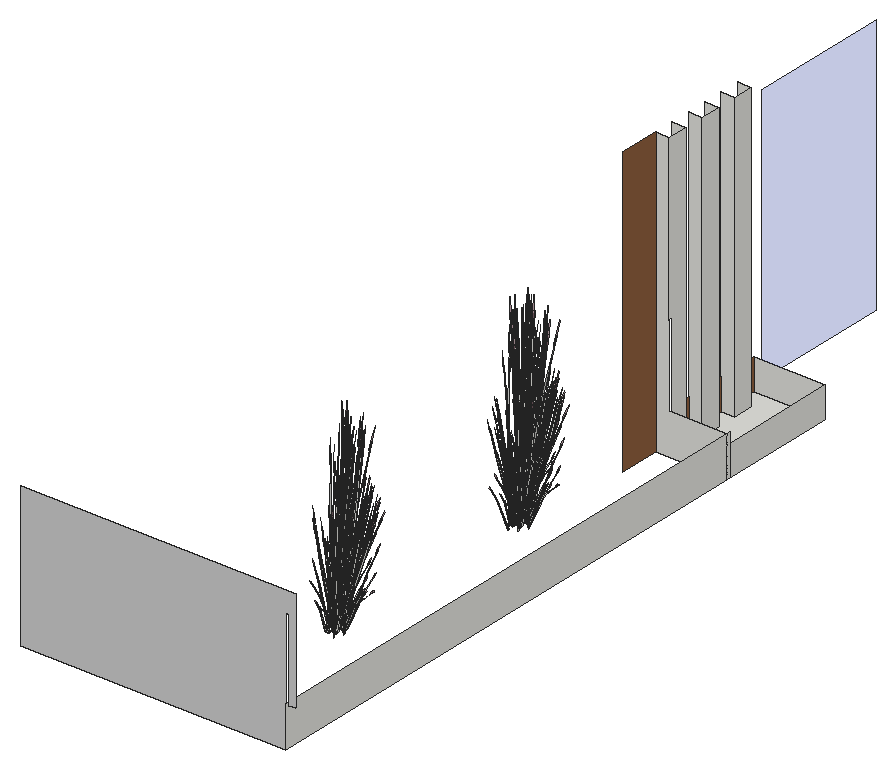
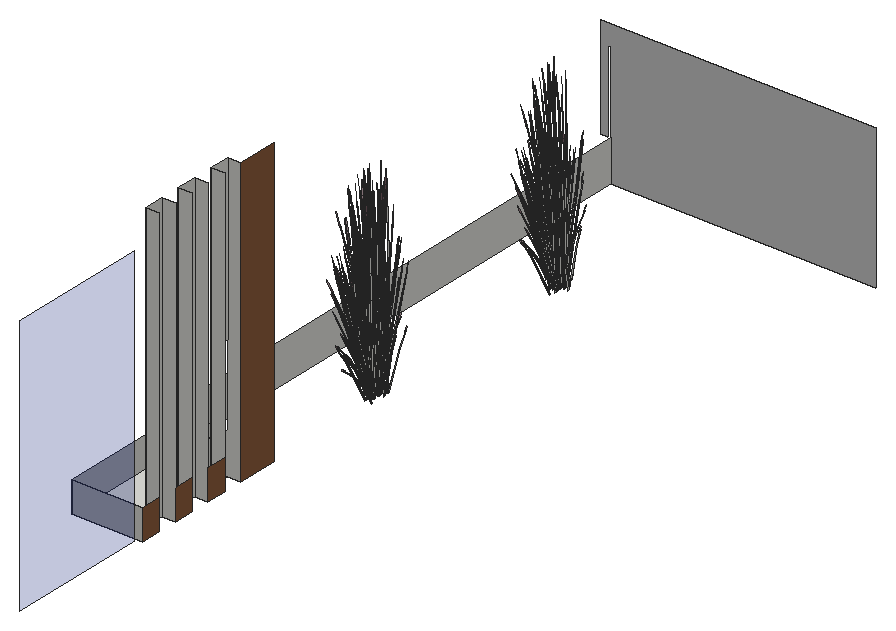
# SketchUp Ruby script. Lengths in inches.
U = 1.inch
M = Sketchup.active_model
def pt(a) = Geom::Point3d.new(a.map { |v| v * U })
def face(e, loops, mat)
  f = e.add_face(loops[0].map { |a| pt(a) })
  loops[1..].each { |l| e.add_face(l.map { |a| pt(a) }).erase! }
  f.material = f.back_material = mat if mat
  f
end
# faces: each face lists its corners as indices into pts; further lists are holes
def faces(e, pts, list, mat = nil) = list.each { |f| face(e, (f[0].is_a?(Array) ? f : [f]).map { |l| l.map { |i| pts[i] } }, mat) }
# xy, xz, yz: faces in a plane at the given z, y or x. An outline is a flat list of corners, or four numbers for a rectangle; further outlines are holes
def ring(l) = l.size == 4 ? [[l[0], l[1]], [l[2], l[1]], [l[2], l[3]], [l[0], l[3]]] : l.each_slice(2).to_a
def flat(e, list, mat, &to3) = list.each { |f| face(e, (f[0].is_a?(Array) ? f : [f]).map { |l| ring(l).map { |u, v| to3.(u, v) } }, mat) }
def xy(e, z, list, mat = nil) = flat(e, list, mat) { |x, y| [x, y, z] }
def xz(e, y, list, mat = nil) = flat(e, list, mat) { |x, z| [x, y, z] }
def yz(e, x, list, mat = nil) = flat(e, list, mat) { |y, z| [x, y, z] }
def lines(e, pts, list) = list.each { |a, b| e.add_line(pt(pts[a]), pt(pts[b])) }
# prism: a flat outline (further loops are holes) pulled along v
def prism(e, loops, v, mat = nil)
  f = face(e, loops, mat); d = Geom::Vector3d.new(v.map { |x| x * U })
  f.pushpull(f.normal.samedirection?(d) ? d.length : -d.length)
end
def box(e, o, s, mat = nil) = prism(e, [[o, [o[0] + s[0], o[1], o[2]], [o[0] + s[0], o[1] + s[1], o[2]], [o[0], o[1] + s[1], o[2]]]], [0, 0, s[2]], mat)
def at(x, y, z, deg = 0) = Geom::Transformation.translation(pt([x, y, z])) * Geom::Transformation.rotation(ORIGIN, Z_AXIS, deg.degrees)
def axes(o, x, y, z) = Geom::Transformation.new([*x, 0, *y, 0, *z, 0, *pt(o).to_a, 1])
def part(name) = M.definitions.add(name)
# library, detail: a bought-in or finely detailed component or shape, given as its bounding box
def library(name, o, s) = part(name).tap { |d| box(d.entities, o, s) }
def detail(e, o, s) = box(e.add_group.entities, o, s)
def put(e, d, t, mat = nil) = e.add_instance(d, t).tap { |i| i.material = mat if mat }
def group(e, t, mat = nil) = e.add_group.tap { |g| g.transformation = t; g.material = mat if mat }.entities
root = M.entities
M.materials.add("Glass_Basic_01").color = [23, 48, 186]
M.materials["Glass_Basic_01"].alpha = 0.25
M.materials.add("LightPink_Translucent").color = [144, 107, 117]
M.materials["LightPink_Translucent"].alpha = 0.75
M.materials.add("Wood_Veneer_15_1K").color = [142, 95, 62]
M.materials.add("[Cladding_Siding_White]1").color = [207, 207, 207]
c1 = part("blade")
p = [[2.15,0.21,22],[0,0.17,0],[0.09,0.45,0],[2.18,0.31,22],[2.29,0.31,22],[0.38,0.45,0],
  [2.48,0.24,33],[2.49,0.24,33],[2.48,0.22,33]]
faces(c1.entities,p,[[0,1,2,3],[4,5,2,3],[6,3,4,7],[8,0,3,6]])
c2 = part("seeds")
p = [[0.3,-0.1,1.38],[-0.01,-0.03,1.59],[-0.01,-0.03,0.03],[0.14,-0.07,-0.07],[0.29,-0.03,3],[0.15,0.01,3.11]]
faces(c2.entities,p,[[0,1,2,3],[1,0,4,5]],"LightPink_Translucent")
c3 = part("blade with seeds")
put(c3.entities,c1,at(0,0,0))
put(c3.entities,c2,axes([2.4,0.25,30.99],[1.5799,-0.05474,1.17369],[-0.12525,1.92788,0.29478],[-0.07173,-0.02425,1.56792]))
xy(root,402,[[364,255,381,256],[364,256,381,256,381,291,360,291,360,285,364,285,364,279,360,279,360,273,364,273,364,267,360,267,360,261,364,261]])
xz(root,93,[[303,402,303,444,384,444,384,414,382,414,382,438,381,438,381,402]],"[Cladding_Siding_White]1")
xz(root,255,[[360,402,381,402,381,414,364,414,364,486,360,486]])
xz(root,256,[[364,402,381,411]])
xz(root,261,[[360,402,364,486]])
xz(root,267,[[360,402,364,486]])
xz(root,273,[[360,402,364,486]])
xz(root,279,[[360,402,364,486]])
xz(root,285,[[360,402,364,486]])
xz(root,291,[[360,402,381,411]])
yz(root,360,[[294,403.5,336,480]],"Glass_Basic_01")
yz(root,360,[[243,402,255,486],[261,402,267,411],[273,402,279,411],[285,402,291,411]],"Wood_Veneer_15_1K")
yz(root,364,[[256,402,261,402,261,486,255,486,255,438,256,438],[267,402,273,486],[279,402,285,486]])
yz(root,381,[[93,402,255,414],[255,402,256,414],[256,402,291,411]])
put(root,c3,axes([357.37,140.09,404.33],[-0.52621,0.16023,0.16584],[-0.12993,-0.59629,0.32981],[0.04693,0.08688,1.50782]))
put(root,c3,axes([356.83,137.86,404.6],[0.06282,0.35202,1.07969],[-0.34848,-0.19497,0.79328],[0.0375,-0.18025,0.23781]))
put(root,c3,axes([356.6,145.46,407.31],[0.3384,-0.34633,-0.06098],[0.31006,0.3793,-0.27651],[0.02183,0.10747,0.91203]))
put(root,c3,axes([356.51,140.96,404.22],[-0.40602,0.54785,0.43009],[-0.48237,-0.48361,0.16877],[0.09788,-0.05467,1.49325]))
put(root,c3,axes([357.2,141.82,404.08],[0.34183,0.38994,0],[-0.34183,0.38994,0],[0,0,1.5911]))
put(root,c3,axes([357.7,208.44,404.33],[0.52621,-0.16023,0.16584],[0.12993,0.59629,0.32981],[-0.04693,-0.08688,1.50782]))
put(root,c3,axes([357.2,141.37,404.56],[0.23759,-0.54397,0.42055],[0.49367,0.26179,-0.2024],[0,0.12539,1.35025]))
put(root,c3,axes([356.99,143.26,404.07],[0.49367,0.27103,0],[-0.23759,0.56315,0],[0,0,1.64456]))
put(root,c3,axes([358.375,208.54,404.0625],[-0.49367,-0.27103,0],[0.23759,-0.56315,0],[0,0,1.52945]))
put(root,c3,axes([358.75,204.62,406.75],[-0.14763,0.46424,0.33289],[-0.4307,-0.1354,-0.42977],[-0.03949,-0.18691,0.82232]))
put(root,c3,axes([359.52,209.22,404.23],[0.30616,0.60492,0],[-0.51222,0.33735,-0.48511],[-0.11666,0.07683,1.53889]))
put(root,c3,axes([356.29,143.98,406.4],[0.48137,0.15133,-0.48033],[-0.165,0.51886,-0.37205],[0.04414,0.2089,0.91906]))
put(root,c3,axes([355.88,144,406.73],[0.47919,-0.28106,-0.11431],[0.23549,0.49884,-0.63445],[0.06322,0.21021,0.96403]))
put(root,c3,axes([357.04,141.24,404.24],[-0.61893,-0.12719,0.46247],[0.12596,-0.71835,0.18148],[0.09045,0.06936,1.60565]))
put(root,c3,axes([357.96,209.48,406.76],[-0.48252,-0.15782,0.50086],[0.165,-0.51886,0.41298],[0.029,0.20404,1.03641]))
put(root,c3,axes([358.33,138.43,406.43],[-0.04973,0.04611,1.6674],[-0.48725,-0.15557,-0.15755],[-0.01764,-0.20123,0.29507]))
put(root,c3,axes([357.94,139.76,406.73],[-0.53819,-0.02991,-0.11431],[0.01471,-0.56632,-0.63445],[0.03738,-0.21811,0.96403]))
put(root,c3,axes([358.45,142.22,403.91],[-0.34183,0.37665,-0.29119],[-0.34183,-0.37665,0.29119],[0,0.12132,1.30635]))
put(root,c3,axes([357.83,209.52,406.45],[-0.36083,0.20517,0.06044],[-0.17661,-0.37413,0.47584],[0.03485,0.16492,0.72558]))
put(root,c3,axes([359.27,208.48,404.33],[0.14146,-0.59996,0.16584],[0.51766,0.16978,0.32981],[-0.08942,0.00292,1.50782]))
put(root,c3,axes([359.03,207.68,404.46],[0.36178,0.36271,0.13611],[-0.30177,0.40921,-0.38866],[-0.084,0.05532,1.1914]))
put(root,c3,axes([357.47,142.15,403.97],[0.17956,0.55272,-0.65059],[-0.51723,0.19906,-0.17075],[0.01985,0.18717,1.43607]))
put(root,c3,axes([357.22,141.56,404.07],[0.54787,0,0],[0,0.62498,0],[0,0,1.67702]))
put(root,c3,axes([358.9,207.23,404.16],[-0.45549,-0.5196,-0.05763],[0.45577,-0.51991,0],[-0.01591,-0.01814,1.65037]))
put(root,c3,axes([357.73,139.85,406.75],[-0.33133,0.31784,0.33289],[-0.31365,-0.36292,-0.42977],[0.04772,-0.1844,0.82232]))
put(root,c3,axes([359.02,207.42,404.56],[0.53176,-0.03727,0.42055],[0.04809,0.6186,-0.2024],[-0.0952,0.0627,1.35025]))
put(root,c3,axes([356.6875,140.87,404.56],[-0.29417,-0.5067,0.42055],[0.44558,-0.35681,-0.2024],[0.0952,0.0627,1.35025]))
put(root,c3,axes([356.15,140.99,404.51],[-0.05706,-0.68884,-0.2735],[0.59432,-0.04165,-0.47002],[0.10465,-0.09176,1.50125]))
put(root,c3,axes([357.41,141.49,404.46],[0.45625,-0.17605,0.13611],[0.15978,0.50273,-0.38866],[0,0.11064,1.1914]))
put(root,c3,axes([357.58,139.55,406.4],[-0.35055,-0.40562,-0.48033],[0.37031,-0.35523,-0.37205],[0.05334,-0.20609,0.91906]))
put(root,c3,axes([359.15,208.84,404.19],[0.61306,0.19622,0.28911],[-0.15337,0.70136,-0.34302],[-0.10147,0.08778,1.54992]))
put(root,c3,axes([358.25,203.46,403.4],[-0.08214,0.02175,1.65762],[-0.45422,-0.24483,-0.25323],[0.00762,-0.20421,0.28235]))
put(root,c3,axes([359.41,208.8,404.33],[0.4583,-0.30184,0.46672],[0.27394,0.54125,0],[-0.10438,0.06875,1.48054]))
put(root,c3,axes([358.7,204.13,406.25],[0.14763,-0.46424,-0.33289],[0.4307,0.1354,0.42977],[-0.03949,-0.18691,0.82232]))
put(root,c3,axes([357.98,206.64,404.22],[0.2129,0.67504,0.43009],[-0.60833,0.23474,0.16877],[0.00743,-0.12404,1.49325]))
put(root,c3,axes([357.25,141.53,404.51],[0.55148,0.28805,-0.2735],[-0.26554,0.60796,-0.47002],[0.01733,0.14927,1.50125]))
put(root,c3,axes([357.88,206.55,404.08],[0.23759,-0.54397,-0.42055],[0.49367,0.26179,0.2024],[0,-0.12539,1.35025]))
put(root,c3,axes([358.49,208.3,404.07],[-0.15978,-0.52046,0],[0.45625,-0.18226,0],[0,0,1.45109]))
put(root,c3,axes([357.91,209.4,403.4],[0.07925,-0.03285,1.65762],[0.47671,0.18081,-0.25323],[0.01394,0.20378,0.28235]))
put(root,c3,axes([356.07,139.46,403.91],[0.45686,0.14937,-0.29119],[-0.11503,0.52602,0.29119],[0.0921,-0.06066,1.30635]))
put(root,c3,axes([358.01,209.59,406.25],[-0.14763,0.46424,-0.33289],[-0.4307,-0.1354,0.42977],[0.03949,0.18691,0.82232]))
put(root,c3,axes([357.35,138.83,404.44],[-0.13919,0.12219,1.34422],[-0.41687,-0.21387,-0.28909],[0.07727,-0.26598,0.57472]))
put(root,c3,axes([358.45,141.67,404.33],[0,-0.60368,0.46672],[0.54787,0,0],[0,0.13749,1.48054]))
put(root,c3,axes([358.68,142.23,403.9],[0,0.60368,-0.46672],[-0.54787,0,0],[0,0.13749,1.48054]))
put(root,c3,axes([357.22,144.0625,406.45],[-0.48705,0.13854,0.45122],[-0.08453,-0.54345,0.37205],[0.11455,0.16017,0.9337]))
put(root,c3,axes([355.97,139.22,403.9],[0.4583,-0.30184,-0.46672],[0.27394,0.54125,0],[0.10438,-0.06875,1.48054]))
put(root,c3,axes([357.125,144.17,406.45],[-0.22256,0.38349,0.06044],[-0.31694,-0.22327,0.47584],[0.10247,0.12295,0.72558]))
put(root,c3,axes([356.5625,142.9,405.64],[-0.11194,-0.19382,1.61094],[0.51725,-0.16318,0.13026],[0.1169,0.30428,0.68866]))
put(root,c3,axes([356.89,140.73,404.46],[0.09447,-0.53876,0.13611],[0.46155,0.09352,-0.38866],[0.084,0.05532,1.1914]))
put(root,c3,axes([359.13,207.28,404.08],[-0.23759,0.54397,-0.42055],[-0.49367,-0.26179,0.2024],[0,0.12539,1.35025]))
put(root,c3,axes([358.88,204.2,406.45],[0.36083,-0.20517,0.06044],[0.17661,0.37413,0.47584],[-0.03485,-0.16492,0.72558]))
put(root,c3,axes([357.71,210.41,406.43],[0.06207,0.09721,1.64448],[0.50093,0.03819,-0.26007],[0.05037,0.21439,0.13189]))
put(root,c3,axes([357.54,139.79,404.33],[-0.4583,-0.30184,0.46672],[0.27394,-0.54125,0],[0.10438,0.06875,1.48054]))
put(root,c3,axes([360.07,206.95,404.33],[-0.38474,-0.43973,0.16584],[0.38772,-0.42651,0.32981],[-0.04249,0.0898,1.50782]))
put(root,c3,axes([357.68,139.73,406.68],[0.01274,-0.55841,-0.66783],[0.53656,0.0375,0.08059],[0.05662,-0.23657,0.9447]))
put(root,c3,axes([358.74,206.69,404.07],[0,-0.69851,0],[0.61233,0,0],[0,0,1.68689]))
put(root,c3,axes([358.75,204.24,406.45],[0.48252,0.15782,0.45122],[-0.165,0.51886,0.37205],[-0.029,-0.20404,0.9337]))
put(root,c3,axes([358.18,206.82,404.29],[0.55175,0.29259,0.22621],[-0.26554,0.60796,0.47002],[0,-0.14015,1.5091]))
put(root,c3,axes([359.05,206.97,404.15],[0,0.69816,-0.05299],[-0.61233,0,0],[0,0.02194,1.68606]))
put(root,c3,axes([358,206.41,404.56],[-0.53176,0.03727,0.42055],[-0.04809,-0.6186,-0.2024],[0.0952,-0.0627,1.35025]))
put(root,c3,axes([357.14,142.9375,404.05],[0.51411,-0.20483,-0.18046],[0.18065,0.59003,0.00007],[0.05675,-0.02264,1.63463]))
put(root,c3,axes([357.97,209.1,406.75],[0.14763,-0.46424,0.33289],[0.4307,0.1354,-0.42977],[0.03949,0.18691,0.82232]))
put(root,c3,axes([357.75,205.35,404.33],[-0.14146,0.59996,0.16584],[-0.51766,-0.16978,0.32981],[0.08942,-0.00292,1.50782]))
put(root,c3,axes([358.76,208.32,404.15],[0.2129,0.69353,-0.05652],[-0.60833,0.24302,0],[0.00743,0.02422,1.61843]))
put(root,c3,axes([357.06,143.73,406.75],[-0.07563,-0.48625,0.33289],[0.43235,-0.1284,-0.42977],[0.11613,0.13934,0.82232]))
put(root,c3,axes([357.15,141.18,404.08],[0.29417,0.5067,-0.42055],[-0.44558,0.35681,0.2024],[0.0952,0.0627,1.35025]))
put(root,c3,axes([357.5,204.61,404.23],[-0.30616,-0.60492,0],[0.51222,-0.33735,-0.48511],[0.11666,-0.07683,1.53889]))
put(root,c3,axes([358.06,209.17,406.68],[0.23372,0.49086,-0.66783],[-0.48111,0.27356,0.08059],[0.05465,0.23717,0.9447]))
put(root,c3,axes([360.52,207.41,404.07],[-0.61202,-0.00483,-0.04678],[0,-0.67471,0.46946],[-0.01923,0.15359,1.48851]))
put(root,c3,axes([357.35,140.93,406.21],[-0.42314,-0.31366,1.29986],[0.4468,-0.48836,0.56085],[0.13652,0.29431,1.25644]))
put(root,c3,axes([357.91,139.4,406.25],[0.33133,-0.31784,-0.33289],[0.31365,0.36292,0.42977],[0.04772,-0.1844,0.82232]))
put(root,c3,axes([356.63,144.41,406.43],[0.00145,-0.07309,1.6674],[0.41965,-0.32245,-0.15755],[0.14577,0.11509,0.29507]))
put(root,c3,axes([358.03,139.5625,406.45],[0.40242,0.02813,0.06044],[-0.01103,0.42474,0.47584],[0.04211,-0.1627,0.72558]))
put(root,c3,axes([359.32,205.38,404.33],[-0.52621,0.16023,0.16584],[-0.12993,-0.59629,0.32981],[0.04693,0.08688,1.50782]))
put(root,c3,axes([357.99,143.48,404.6],[-0.27572,-0.17358,1.07969],[0.35602,-0.17637,0.79328],[0.09603,0.1494,0.23781]))
put(root,c3,axes([357,143.3,404.44],[0.00864,-0.20012,1.34422],[0.41296,-0.22353,-0.28909],[0.12748,0.23952,0.57472]))
put(root,c3,axes([358.43,138.86,406.43],[-0.00473,-0.12015,1.64448],[-0.39924,-0.34724,-0.26007],[0.06173,-0.21049,0.13189]))
put(root,c3,axes([356.51,140.46,403.9375],[0.32983,-0.45375,-0.58612],[0.40974,0.41145,-0.15383],[0.13217,-0.11319,1.29375]))
put(root,c3,axes([358.78,203.15,404.6],[0.06282,0.35202,1.07969],[-0.34848,-0.19497,0.79328],[0.0375,-0.18025,0.23781]))
put(root,c3,axes([358.55,210.75,407.31],[0.3384,-0.34633,-0.06098],[0.31006,0.3793,-0.27651],[0.02183,0.10747,0.91203]))
put(root,c3,axes([357.9,139.52,406.45],[0.3487,0.41189,0.45122],[-0.37031,0.35523,0.37205],[0.06432,-0.19325,0.9337]))
put(root,c3,axes([358.45,206.25,404.22],[-0.40602,0.54785,0.43009],[-0.48237,-0.48361,0.16877],[0.09788,-0.05467,1.49325]))
put(root,c3,axes([359.15,207.12,404.08],[0.34183,0.38994,0],[-0.34183,0.38994,0],[0,0,1.5911]))
put(root,c3,axes([359.14,206.66,404.56],[0.23759,-0.54397,0.42055],[0.49367,0.26179,-0.2024],[0,0.12539,1.35025]))
put(root,c3,axes([358.9375,208.55,404.07],[0.49367,0.27103,0],[-0.23759,0.56315,0],[0,0,1.64456]))
put(root,c3,axes([358.23,209.27,406.4],[0.48137,0.15133,-0.48033],[-0.165,0.51886,-0.37205],[0.04414,0.2089,0.91906]))
put(root,c3,axes([357.96,140.06,403.91],[0.11503,0.52602,-0.29119],[-0.45686,0.14937,0.29119],[0.0921,0.06066,1.30635]))
put(root,c3,axes([358.82,141.77,404.23],[0.61233,0,0],[0,0.67471,-0.48511],[0,0.15367,1.53889]))
put(root,c3,axes([357.82,209.29,406.73],[0.47919,-0.28106,-0.11431],[0.23549,0.49884,-0.63445],[0.06322,0.21021,0.96403]))
put(root,c3,axes([358.98,206.53,404.24],[-0.61893,-0.12719,0.46247],[0.12596,-0.71835,0.18148],[0.09045,0.06936,1.60565]))
put(root,c3,axes([360.27,203.72,406.43],[-0.04973,0.04611,1.6674],[-0.48725,-0.15557,-0.15755],[-0.01764,-0.20123,0.29507]))
put(root,c3,axes([359.89,205.05,406.73],[-0.53819,-0.02991,-0.11431],[0.01471,-0.56632,-0.63445],[0.03738,-0.21811,0.96403]))
put(root,c3,axes([360.39,207.51,403.91],[-0.34183,0.37665,-0.29119],[-0.34183,-0.37665,0.29119],[0,0.12132,1.30635]))
put(root,c3,axes([356.84,140.9,404.51],[0.49442,-0.40079,-0.2735],[0.32878,0.56631,-0.47002],[0.12199,0.05751,1.50125]))
put(root,c3,axes([358.03,144.27,404.51],[-0.31402,-0.01893,0.98757],[0.20738,-0.40212,0.54525],[0.12405,0.14286,0.77466]))
put(root,c3,axes([358.31,140.83,406.75],[-0.42626,0.08628,0.33289],[-0.11256,-0.4932,-0.42977],[0.12215,-0.13247,0.82232]))
put(root,c3,axes([359.41,207.44,403.97],[0.17956,0.55272,-0.65059],[-0.51723,0.19906,-0.17075],[0.01985,0.18717,1.43607]))
put(root,c3,axes([359.16,206.85,404.07],[0.54787,0,0],[0,0.62498,0],[0,0,1.67702]))
put(root,c3,axes([357.08,139.45,405.64],[-0.09118,0.2075,1.61094],[-0.3825,-0.42941,0.13026],[0.17255,-0.26763,0.68866]))
put(root,c3,axes([359.68,205.14,406.75],[-0.33133,0.31784,0.33289],[-0.31365,-0.36292,-0.42977],[0.04772,-0.1844,0.82232]))
put(root,c3,axes([358.63,206.16,404.56],[-0.29417,-0.5067,0.42055],[0.44558,-0.35681,-0.2024],[0.0952,0.0627,1.35025]))
put(root,c3,axes([358.1,206.28,404.51],[-0.05706,-0.68884,-0.2735],[0.59432,-0.04165,-0.47002],[0.10465,-0.09176,1.50125]))
put(root,c3,axes([359.35,206.79,404.46],[0.45625,-0.17605,0.13611],[0.15978,0.50273,-0.38866],[0,0.11064,1.1914]))
put(root,c3,axes([359.52,204.84,406.4],[-0.35055,-0.40562,-0.48033],[0.37031,-0.35523,-0.37205],[0.05334,-0.20609,0.91906]))
put(root,c3,axes([357.02,143.98,406.73],[0.2918,-0.51673,-0.11431],[0.42258,0.29769,-0.63445],[0.14689,0.14599,0.96403]))
put(root,c3,axes([355.59,140.54,403.5],[-0.482,0.24169,1.21193],[-0.15342,-0.69348,0.47091],[0.29598,0.01154,1.37843]))
put(root,c3,axes([358.53,140.875,406.73],[-0.45297,-0.33287,-0.11431],[0.26096,-0.48206,-0.63445],[0.12798,-0.16757,0.96403]))
put(root,c3,axes([359.19,206.83,404.51],[0.55148,0.28805,-0.2735],[-0.26554,0.60796,-0.47002],[0.01733,0.14927,1.50125]))
put(root,c3,axes([358.02,204.76,403.91],[0.45686,0.14937,-0.29119],[-0.11503,0.52602,0.29119],[0.0921,-0.06066,1.30635]))
put(root,c3,axes([359.29,204.12,404.44],[-0.13919,0.12219,1.34422],[-0.41687,-0.21387,-0.28909],[0.07727,-0.26598,0.57472]))
put(root,c3,axes([357.36,143.72,406.4],[0.48321,-0.1435,-0.48033],[0.08453,0.54345,-0.37205],[0.12979,0.15574,0.91906]))
put(root,c3,axes([357.81,139.47,404.23],[0.30616,-0.60492,0],[0.51222,0.33735,-0.48511],[0.11666,0.07683,1.53889]))
put(root,c3,axes([358.32,139.21,403.4],[-0.07329,-0.04756,1.65762],[-0.18827,-0.53132,-0.25323],[0.127,-0.14418,0.28235]))
put(root,c3,axes([360.39,206.96,404.33],[0,-0.60368,0.46672],[0.54787,0,0],[0,0.13749,1.48054]))
put(root,c3,axes([357.92,143.07,406.75],[-0.27863,-0.37797,0.33289],[0.31815,-0.35779,-0.42977],[0.16164,0.05444,0.82232]))
put(root,c3,axes([360.625,207.52,403.9],[0,0.60368,-0.46672],[-0.54787,0,0],[0,0.13749,1.48054]))
put(root,c3,axes([359.16,209.35,406.45],[-0.48705,0.13854,0.45122],[-0.08453,-0.54345,0.37205],[0.11455,0.16017,0.9337]))
put(root,c3,axes([357.91,204.52,403.9],[0.4583,-0.30184,-0.46672],[0.27394,0.54125,0],[0.10438,-0.06875,1.48054]))
put(root,c3,axes([359.07,209.46,406.45],[-0.22256,0.38349,0.06044],[-0.31694,-0.22327,0.47584],[0.10247,0.12295,0.72558]))
put(root,c3,axes([358.51,208.2,405.64],[-0.11194,-0.19382,1.61094],[0.51725,-0.16318,0.13026],[0.1169,0.30428,0.68866]))
put(root,c3,axes([358.09,139.83,403.9],[0.4583,0.30184,-0.46672],[-0.27394,0.54125,0],[0.10438,0.06875,1.48054]))
put(root,c3,axes([358.83,206.02,404.46],[0.09447,-0.53876,0.13611],[0.46155,0.09352,-0.38866],[0.084,0.05532,1.1914]))
put(root,c3,axes([358.17,143.41,406.45],[-0.02466,0.45905,0.06044],[-0.37234,-0.01259,0.47584],[0.14263,0.04803,0.72558]))
put(root,c3,axes([358.0625,144.13,403.4],[0.03568,-0.08715,1.65762],[0.44916,-0.25668,-0.25323],[0.13617,0.13285,0.28235]))
put(root,c3,axes([358.2,143.27,406.45],[-0.36108,0.39778,0.45122],[-0.31141,-0.42243,0.37205],[0.1694,0.07337,0.9337]))
put(root,c3,axes([358.3,140.48,406.4],[-0.1258,-0.55122,-0.48033],[0.4764,-0.09643,-0.37205],[0.13652,-0.14806,0.91906]))
put(root,c3,axes([359.49,205.08,404.33],[-0.4583,-0.30184,0.46672],[0.27394,-0.54125,0],[0.10438,0.06875,1.48054]))
put(root,c3,axes([359.14,143.33,405.69],[-0.09372,-0.50747,-0.03282],[0.44299,-0.11666,-0.14882],[0.09251,0.03217,0.49085]))
put(root,c3,axes([358.375,142.01,406.75],[-0.40696,-0.16841,0.33289],[0.1187,-0.49132,-0.42977],[0.16385,-0.04505,0.82232]))
put(root,c3,axes([359.63,205.03,406.68],[0.01274,-0.55841,-0.66783],[0.53656,0.0375,0.08059],[0.05662,-0.23657,0.9447]))
put(root,c3,axes([357.42,140.99,403.9375],[0.50939,0.09897,-0.58612],[-0.10749,0.61051,-0.15383],[0.15202,0.07398,1.29375]))
put(root,c3,axes([359.09,208.23,404.05],[0.51411,-0.20483,-0.18046],[0.18065,0.59003,0.00007],[0.05675,-0.02264,1.63463]))
put(root,c3,axes([359.59,141.35,404.125],[-0.3036,-0.38602,-0.06098],[0.3325,-0.3537,-0.27651],[0.09421,-0.0249,0.91203]))
put(root,c3,axes([358.89,139.39,404.6],[-0.16311,0.3073,1.07969],[-0.1402,-0.41288,0.79328],[0.13471,-0.10346,0.23781]))
put(root,c3,axes([359,209.02,406.75],[-0.07563,-0.48625,0.33289],[0.43235,-0.1284,-0.42977],[0.11613,0.13934,0.82232]))
put(root,c3,axes([358.69,140.75,406.45],[0.33617,0.25389,0.06044],[-0.19572,0.36154,0.47584],[0.10778,-0.11689,0.72558]))
put(root,c3,axes([359.1,206.48,404.08],[0.29417,0.5067,-0.42055],[-0.44558,0.35681,0.2024],[0.0952,0.0627,1.35025]))
put(root,c3,axes([358.6,140.65,406.45],[0.12145,0.5556,0.45122],[-0.4764,0.09643,0.37205],[0.14041,-0.13067,0.9337]))
put(root,c3,axes([359.29,206.22,406.21],[-0.42314,-0.31366,1.29986],[0.4468,-0.48836,0.56085],[0.13652,0.29431,1.25644]))
put(root,c3,axes([359.85,204.69,406.25],[0.33133,-0.31784,-0.33289],[0.31365,0.36292,0.42977],[0.04772,-0.1844,0.82232]))
put(root,c3,axes([358.58,209.7,406.43],[0.00145,-0.07309,1.6674],[0.41965,-0.32245,-0.15755],[0.14577,0.11509,0.29507]))
put(root,c3,axes([359.98,204.85,406.45],[0.40242,0.02813,0.06044],[-0.01103,0.42474,0.47584],[0.04211,-0.1627,0.72558]))
put(root,c3,axes([359.93,208.78,404.6],[-0.27572,-0.17358,1.07969],[0.35602,-0.17637,0.79328],[0.09603,0.1494,0.23781]))
put(root,c3,axes([358.95,208.59,404.44],[0.00864,-0.20012,1.34422],[0.41296,-0.22353,-0.28909],[0.12748,0.23952,0.57472]))
put(root,c3,axes([357.3125,142.3,405.64],[-0.1819,-0.10401,1.61094],[0.37643,-0.43634,0.13026],[0.23461,0.19684,0.68866]))
put(root,c3,axes([360.38,204.15,406.43],[-0.00473,-0.12015,1.64448],[-0.39924,-0.34724,-0.26007],[0.06173,-0.21049,0.13189]))
put(root,c3,axes([358.46,205.76,403.9375],[0.32983,-0.45375,-0.58612],[0.40974,0.41145,-0.15383],[0.13217,-0.11319,1.29375]))
put(root,c3,axes([359.64,140.73,406.43],[-0.06396,-0.00458,1.6674],[-0.2656,-0.49127,-0.15755],[0.10666,-0.16153,0.29507]))
put(root,c3,axes([359.85,204.81,406.45],[0.3487,0.41189,0.45122],[-0.37031,0.35523,0.37205],[0.06432,-0.19325,0.9337]))
put(root,c3,axes([358.66,140.54,406.25],[0.42626,-0.08628,-0.33289],[0.11256,0.4932,0.42977],[0.12215,-0.13247,0.82232]))
put(root,c3,axes([358.32,140.7,406.68],[0.25579,-0.47633,-0.66783],[0.44823,0.33852,0.08059],[0.15273,-0.17258,0.9447]))
put(root,c3,axes([358.74,142.16,406.45],[0.17985,0.41162,0.06044],[-0.32797,0.20147,0.47584],[0.14457,-0.03975,0.72558]))
put(root,c3,axes([358.3125,143.27,406.25],[0.27863,0.37797,-0.33289],[-0.31815,0.35779,0.42977],[0.16164,0.05444,0.82232]))
put(root,c3,axes([357.99,143.3125,406.73],[0.02622,-0.61393,-0.11431],[0.49645,0.01678,-0.63445],[0.1912,0.04265,0.96403]))
put(root,c3,axes([358.55,142.18,406.73],[-0.24639,-0.54664,-0.11431],[0.43729,-0.26863,-0.63445],[0.18428,-0.07212,0.96403]))
put(root,c3,axes([359.9,205.35,403.91],[0.11503,0.52602,-0.29119],[-0.45686,0.14937,0.29119],[0.0921,0.06066,1.30635]))
put(root,c3,axes([360.76,207.07,404.23],[0.61233,0,0],[0,0.67471,-0.48511],[0,0.15367,1.53889]))
put(root,c3,axes([358.71,142.02,406.45],[-0.13835,0.55043,0.45122],[-0.45484,-0.18822,0.37205],[0.17887,-0.03308,0.9337]))
put(root,c3,axes([358.78,206.19,404.51],[0.49442,-0.40079,-0.2735],[0.32878,0.56631,-0.47002],[0.12199,0.05751,1.50125]))
put(root,c3,axes([359.97,209.57,404.51],[-0.31402,-0.01893,0.98757],[0.20738,-0.40212,0.54525],[0.12405,0.14286,0.77466]))
put(root,c3,axes([360.25,206.125,406.75],[-0.42626,0.08628,0.33289],[-0.11256,-0.4932,-0.42977],[0.12215,-0.13247,0.82232]))
put(root,c3,axes([359.03,204.74,405.64],[-0.09118,0.2075,1.61094],[-0.3825,-0.42941,0.13026],[0.17255,-0.26763,0.68866]))
put(root,c3,axes([358.43,142.94,406.43],[0.10505,-0.01021,1.64448],[0.28813,-0.469,-0.26007],[0.18685,0.06191,0.13189]))
put(root,c3,axes([358.53,141.71,406.4],[0.13266,-0.54912,-0.48033],[0.45484,0.18822,-0.37205],[0.18313,-0.05035,0.91906]))
put(root,c3,axes([358.96,209.27,406.73],[0.2918,-0.51673,-0.11431],[0.42258,0.29769,-0.63445],[0.14689,0.14599,0.96403]))
put(root,c3,axes([359.67,142.06,404.6],[-0.30256,0.09966,1.07969],[0.14242,-0.41189,0.79328],[0.16051,0.02818,0.23781]))
put(root,c3,axes([357.54,205.84,403.5],[-0.482,0.24169,1.21193],[-0.15342,-0.69348,0.47091],[0.29598,0.01154,1.37843]))
put(root,c3,axes([360.47,206.17,406.73],[-0.45297,-0.33287,-0.11431],[0.26096,-0.48206,-0.63445],[0.12798,-0.16757,0.96403]))
put(root,c3,axes([358.6875,140.27,404.44],[-0.17494,-0.01788,1.34422],[-0.17922,-0.47967,-0.28909],[0.21491,-0.13569,0.57472]))
put(root,c3,axes([358.8,141.96,406.25],[0.40696,0.16841,-0.33289],[-0.1187,0.49132,0.42977],[0.16385,-0.04505,0.82232]))
put(root,c3,axes([359.31,209.02,406.4],[0.48321,-0.1435,-0.48033],[0.08453,0.54345,-0.37205],[0.12979,0.15574,0.91906]))
put(root,c3,axes([359.75,204.76,404.23],[0.30616,-0.60492,0],[0.51222,0.33735,-0.48511],[0.11666,0.07683,1.53889]))
put(root,c3,axes([360.26,204.5,403.4],[-0.07329,-0.04756,1.65762],[-0.18827,-0.53132,-0.25323],[0.127,-0.14418,0.28235]))
put(root,c3,axes([359.86,208.36,406.75],[-0.27863,-0.37797,0.33289],[0.31815,-0.35779,-0.42977],[0.16164,0.05444,0.82232]))
put(root,c3,axes([358.02,143.02,406.68],[0.48951,0.01454,-0.66783],[-0.03288,0.61207,0.08059],[0.20738,0.06459,0.9447]))
put(root,c3,axes([360.03,205.13,403.9],[0.4583,0.30184,-0.46672],[-0.27394,0.54125,0],[0.10438,0.06875,1.48054]))
put(root,c3,axes([359.01,141.86,403.86],[-0.3154,0.07245,1.33088],[-0.0502,-0.57666,0.07618],[0.2209,-0.08728,0.75732]))
put(root,c3,axes([360.11,208.71,406.45],[-0.02466,0.45905,0.06044],[-0.37234,-0.01259,0.47584],[0.14263,0.04803,0.72558]))
put(root,c3,axes([359.36,141.48,403.4],[-0.02559,-0.09165,1.65762],[0.1775,-0.53611,-0.25323],[0.17905,-0.00771,0.28235]))
put(root,c3,axes([360.01,209.42,403.4],[0.03568,-0.08715,1.65762],[0.44916,-0.25668,-0.25323],[0.13617,0.13285,0.28235]))
put(root,c3,axes([360.15,208.56,406.45],[-0.36108,0.39778,0.45122],[-0.31141,-0.42243,0.37205],[0.1694,0.07337,0.9337]))
put(root,c3,axes([360.25,205.77,406.4],[-0.1258,-0.55122,-0.48033],[0.4764,-0.09643,-0.37205],[0.13652,-0.14806,0.91906]))
put(root,c3,axes([359.53,143.8,406.43],[-0.04428,-0.05285,1.6674],[0.09686,-0.56651,-0.15755],[0.17442,-0.03619,0.29507]))
put(root,c3,axes([357.7,141.35,405.64],[-0.20312,0.01367,1.61094],[0.13474,-0.59258,0.13026],[0.28946,0.03665,0.68866]))
put(root,c3,axes([361.09,208.62,405.69],[-0.09372,-0.50747,-0.03282],[0.44299,-0.11666,-0.14882],[0.09251,0.03217,0.49085]))
put(root,c3,axes([360.32,207.3,406.75],[-0.40696,-0.16841,0.33289],[0.1187,-0.49132,-0.42977],[0.16385,-0.04505,0.82232]))
put(root,c3,axes([359.36,206.28,403.9375],[0.50939,0.09897,-0.58612],[-0.10749,0.61051,-0.15383],[0.15202,0.07398,1.29375]))
put(root,c3,axes([361.53,206.64,404.125],[-0.3036,-0.38602,-0.06098],[0.3325,-0.3537,-0.27651],[0.09421,-0.0249,0.91203]))
put(root,c3,axes([358.4375,141.91,406.68],[0.4303,-0.26662,-0.66783],[0.23981,0.54882,0.08059],[0.20791,-0.06234,0.9447]))
put(root,c3,axes([360.83,204.68,404.6],[-0.16311,0.3073,1.07969],[-0.1402,-0.41288,0.79328],[0.13471,-0.10346,0.23781]))
put(root,c3,axes([360.64,206.05,406.45],[0.33617,0.25389,0.06044],[-0.19572,0.36154,0.47584],[0.10778,-0.11689,0.72558]))
put(root,c3,axes([359.89,141.32,406.43],[0.06795,-0.09195,1.64448],[-0.08698,-0.56405,-0.26007],[0.1705,-0.10694,0.13189]))
put(root,c3,axes([360.54,205.9375,406.45],[0.12145,0.5556,0.45122],[-0.4764,0.09643,0.37205],[0.14041,-0.13067,0.9337]))
put(root,c3,axes([359.1,142.72,404.44],[-0.11793,-0.14847,1.34422],[0.15345,-0.49116,-0.28909],[0.23861,0.06653,0.57472]))
put(root,c3,axes([359.26,207.59,405.64],[-0.1819,-0.10401,1.61094],[0.37643,-0.43634,0.13026],[0.23461,0.19684,0.68866]))
put(root,c3,axes([361.59,206.02,406.43],[-0.06396,-0.00458,1.6674],[-0.2656,-0.49127,-0.15755],[0.10666,-0.16153,0.29507]))
put(root,c3,axes([360.6,205.83,406.25],[0.42626,-0.08628,-0.33289],[0.11256,0.4932,0.42977],[0.12215,-0.13247,0.82232]))
put(root,c3,axes([360.26,206,406.68],[0.25579,-0.47633,-0.66783],[0.44823,0.33852,0.08059],[0.15273,-0.17258,0.9447]))
put(root,c3,axes([360.6875,207.46,406.45],[0.17985,0.41162,0.06044],[-0.32797,0.20147,0.47584],[0.14457,-0.03975,0.72558]))
put(root,c3,axes([360.26,208.5625,406.25],[0.27863,0.37797,-0.33289],[-0.31815,0.35779,0.42977],[0.16164,0.05444,0.82232]))
put(root,c3,axes([359.9375,208.6,406.73],[0.02622,-0.61393,-0.11431],[0.49645,0.01678,-0.63445],[0.1912,0.04265,0.96403]))
put(root,c3,axes([360.49,207.47,406.73],[-0.24639,-0.54664,-0.11431],[0.43729,-0.26863,-0.63445],[0.18428,-0.07212,0.96403]))
put(root,c3,axes([360.65,207.31,406.45],[-0.13835,0.55043,0.45122],[-0.45484,-0.18822,0.37205],[0.17887,-0.03308,0.9337]))
put(root,c3,axes([360.37,208.24,406.43],[0.10505,-0.01021,1.64448],[0.28813,-0.469,-0.26007],[0.18685,0.06191,0.13189]))
put(root,c3,axes([360.47,207,406.4],[0.13266,-0.54912,-0.48033],[0.45484,0.18822,-0.37205],[0.18313,-0.05035,0.91906]))
put(root,c3,axes([361.61,207.35,404.6],[-0.30256,0.09966,1.07969],[0.14242,-0.41189,0.79328],[0.16051,0.02818,0.23781]))
put(root,c3,axes([360.63,205.56,404.44],[-0.17494,-0.01788,1.34422],[-0.17922,-0.47967,-0.28909],[0.21491,-0.13569,0.57472]))
put(root,c3,axes([360.75,207.25,406.25],[0.40696,0.16841,-0.33289],[-0.1187,0.49132,0.42977],[0.16385,-0.04505,0.82232]))
put(root,c3,axes([359.96,208.31,406.68],[0.48951,0.01454,-0.66783],[-0.03288,0.61207,0.08059],[0.20738,0.06459,0.9447]))
put(root,c3,axes([360.96,207.15,403.86],[-0.3154,0.07245,1.33088],[-0.0502,-0.57666,0.07618],[0.2209,-0.08728,0.75732]))
put(root,c3,axes([361.3,206.78,403.4],[-0.02559,-0.09165,1.65762],[0.1775,-0.53611,-0.25323],[0.17905,-0.00771,0.28235]))
put(root,c3,axes([361.47,209.09,406.43],[-0.04428,-0.05285,1.6674],[0.09686,-0.56651,-0.15755],[0.17442,-0.03619,0.29507]))
put(root,c3,axes([359.64,206.64,405.64],[-0.20312,0.01367,1.61094],[0.13474,-0.59258,0.13026],[0.28946,0.03665,0.68866]))
put(root,c3,axes([360.38,207.2,406.68],[0.4303,-0.26662,-0.66783],[0.23981,0.54882,0.08059],[0.20791,-0.06234,0.9447]))
put(root,c3,axes([361.83,206.61,406.43],[0.06795,-0.09195,1.64448],[-0.08698,-0.56405,-0.26007],[0.1705,-0.10694,0.13189]))
put(root,c3,axes([361.05,208.01,404.44],[-0.11793,-0.14847,1.34422],[0.15345,-0.49116,-0.28909],[0.23861,0.06653,0.57472]))
